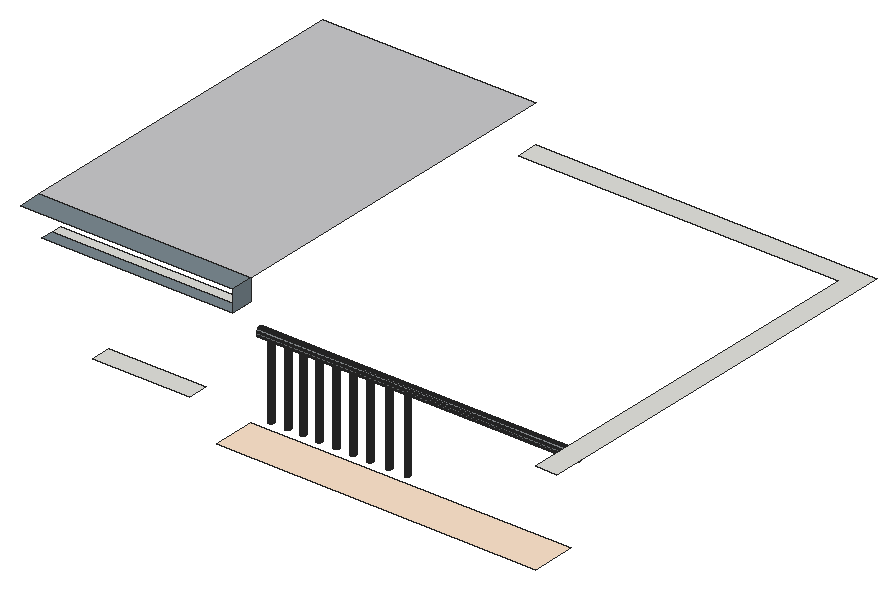
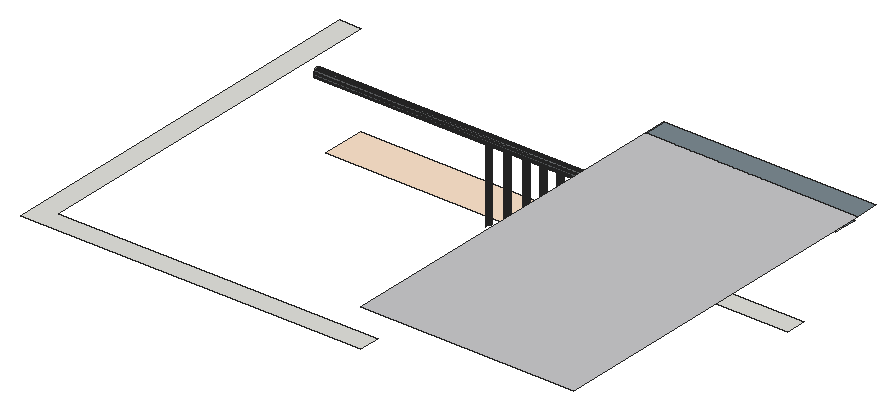
# SketchUp Ruby script. Lengths in inches.
U = 1.inch
M = Sketchup.active_model
def pt(a) = Geom::Point3d.new(a.map { |v| v * U })
def face(e, loops, mat)
  f = e.add_face(loops[0].map { |a| pt(a) })
  loops[1..].each { |l| e.add_face(l.map { |a| pt(a) }).erase! }
  f.material = f.back_material = mat if mat
  f
end
# faces: each face lists its corners as indices into pts; further lists are holes
def faces(e, pts, list, mat = nil) = list.each { |f| face(e, (f[0].is_a?(Array) ? f : [f]).map { |l| l.map { |i| pts[i] } }, mat) }
# xy, xz, yz: faces in a plane at the given z, y or x. An outline is a flat list of corners, or four numbers for a rectangle; further outlines are holes
def ring(l) = l.size == 4 ? [[l[0], l[1]], [l[2], l[1]], [l[2], l[3]], [l[0], l[3]]] : l.each_slice(2).to_a
def flat(e, list, mat, &to3) = list.each { |f| face(e, (f[0].is_a?(Array) ? f : [f]).map { |l| ring(l).map { |u, v| to3.(u, v) } }, mat) }
def xy(e, z, list, mat = nil) = flat(e, list, mat) { |x, y| [x, y, z] }
def xz(e, y, list, mat = nil) = flat(e, list, mat) { |x, z| [x, y, z] }
def yz(e, x, list, mat = nil) = flat(e, list, mat) { |y, z| [x, y, z] }
def lines(e, pts, list) = list.each { |a, b| e.add_line(pt(pts[a]), pt(pts[b])) }
# prism: a flat outline (further loops are holes) pulled along v
def prism(e, loops, v, mat = nil)
  f = face(e, loops, mat); d = Geom::Vector3d.new(v.map { |x| x * U })
  f.pushpull(f.normal.samedirection?(d) ? d.length : -d.length)
end
def box(e, o, s, mat = nil) = prism(e, [[o, [o[0] + s[0], o[1], o[2]], [o[0] + s[0], o[1] + s[1], o[2]], [o[0], o[1] + s[1], o[2]]]], [0, 0, s[2]], mat)
def at(x, y, z, deg = 0) = Geom::Transformation.translation(pt([x, y, z])) * Geom::Transformation.rotation(ORIGIN, Z_AXIS, deg.degrees)
def axes(o, x, y, z) = Geom::Transformation.new([*x, 0, *y, 0, *z, 0, *pt(o).to_a, 1])
def part(name) = M.definitions.add(name)
# library, detail: a bought-in or finely detailed component or shape, given as its bounding box
def library(name, o, s) = part(name).tap { |d| box(d.entities, o, s) }
def detail(e, o, s) = box(e.add_group.entities, o, s)
def put(e, d, t, mat = nil) = e.add_instance(d, t).tap { |i| i.material = mat if mat }
def group(e, t, mat = nil) = e.add_group.tap { |g| g.transformation = t; g.material = mat if mat }.entities
root = M.entities
M.materials.add("[Blacktop Old 01]").color = [132, 136, 139]
M.materials.add("[Color C01]").color = [255, 229, 204]
M.materials.add("[Formica Speckled Grey]").color = [123, 137, 145]
M.materials.add("[Polished Concrete New]").color = [200, 200, 203]
M.materials.add("[Terrazzo Light Blue]").color = [196, 214, 227]
xy(root,2196.1875,[[746.18,617.28,1870.17,769.97]],"[Color C01]")
xy(root,2229.35,[[218.87,733.78,559.3,805.03]])
xy(root,2459.4375,[[1199.35,798.92,1201.92,799.26,1204.32,800.25,1206.375,801.83,1207.95,803.89,1208.95,806.29,1209.29,808.86,1208.95,811.43,1207.95,813.83,1206.375,815.89,1204.32,817.46,1201.92,818.46,1199.35,818.8,1196.78,818.46,1194.38,817.46,1192.32,815.89,1190.74,813.83,1189.75,811.43,1189.41,808.86,1189.75,806.29,1190.74,803.89,1192.32,801.83,1194.38,800.25,1196.78,799.26]])
xy(root,2460.4375,[[1524.85,798.92,1527.42,799.26,1529.82,800.25,1531.875,801.83,1533.45,803.89,1534.45,806.29,1534.79,808.86,1534.45,811.43,1533.45,813.83,1531.875,815.89,1529.82,817.46,1527.42,818.46,1524.85,818.8,1522.28,818.46,1519.88,817.46,1517.82,815.89,1516.24,813.83,1515.25,811.43,1514.91,808.86,1515.25,806.29,1516.24,803.89,1517.82,801.83,1519.88,800.25,1522.28,799.26]])
xy(root,2461.125,[[1396.47,798.92,1399.05,799.26,1401.44,800.25,1403.5,801.83,1405.08,803.89,1406.07,806.29,1406.41,808.86,1406.07,811.43,1405.08,813.83,1403.5,815.89,1401.44,817.46,1399.05,818.46,1396.47,818.8,1393.9,818.46,1391.5,817.46,1389.45,815.89,1387.87,813.83,1386.875,811.43,1386.54,808.86,1386.875,806.29,1387.87,803.89,1389.45,801.83,1391.5,800.25,1393.9,799.26]])
xy(root,2462.0625,[[954.66,798.92,957.23,799.26,959.63,800.25,961.6875,801.83,963.27,803.89,964.26,806.29,964.6,808.86,964.26,811.43,963.27,813.83,961.6875,815.89,959.63,817.46,957.23,818.46,954.66,818.8,952.09,818.46,949.69,817.46,947.63,815.89,946.06,813.83,945.0625,811.43,944.72,808.86,945.0625,806.29,946.06,803.89,947.63,801.83,949.69,800.25,952.09,799.26]])
xy(root,2462.1875,[[1135.1,798.92,1137.67,799.26,1140.07,800.25,1142.125,801.83,1143.7,803.89,1144.7,806.29,1145.04,808.86,1144.7,811.43,1143.7,813.83,1142.125,815.89,1140.07,817.46,1137.67,818.46,1135.1,818.8,1132.53,818.46,1130.13,817.46,1128.07,815.89,1126.49,813.83,1125.5,811.43,1125.16,808.86,1125.5,806.29,1126.49,803.89,1128.07,801.83,1130.13,800.25,1132.53,799.26]])
xy(root,2464.4375,[[1644.29,798.92,1646.86,799.26,1649.25,800.25,1651.3125,801.83,1652.89,803.89,1653.89,806.29,1654.22,808.86,1653.89,811.43,1652.89,813.83,1651.3125,815.89,1649.25,817.46,1646.86,818.46,1644.29,818.8,1641.71,818.46,1639.32,817.46,1637.26,815.89,1635.68,813.83,1634.6875,811.43,1634.35,808.86,1634.6875,806.29,1635.68,803.89,1637.26,801.83,1639.32,800.25,1641.71,799.26]])
xy(root,2464.74,[[1015.1,798.92,1017.67,799.26,1020.07,800.25,1022.125,801.83,1023.7,803.89,1024.7,806.29,1025.04,808.86,1024.7,811.43,1023.7,813.83,1022.125,815.89,1020.07,817.46,1017.67,818.46,1015.1,818.8,1012.53,818.46,1010.13,817.46,1008.07,815.89,1006.49,813.83,1005.5,811.43,1005.16,808.86,1005.5,806.29,1006.49,803.89,1008.07,801.83,1010.13,800.25,1012.53,799.26],[1760.72,798.92,1763.3,799.26,1765.69,800.25,1767.75,801.83,1769.33,803.89,1770.32,806.29,1770.66,808.86,1770.32,811.43,1769.33,813.83,1767.75,815.89,1765.69,817.46,1763.3,818.46,1760.72,818.8,1758.15,818.46,1755.75,817.46,1753.7,815.89,1752.12,813.83,1751.125,811.43,1750.79,808.86,1751.125,806.29,1752.12,803.89,1753.7,801.83,1755.75,800.25,1758.15,799.26]])
xy(root,2466.1875,[[1705.97,798.92,1708.55,799.26,1710.94,800.25,1713,801.83,1714.58,803.89,1715.57,806.29,1715.91,808.86,1715.57,811.43,1714.58,813.83,1713,815.89,1710.94,817.46,1708.55,818.46,1705.97,818.8,1703.4,818.46,1701,817.46,1698.95,815.89,1697.37,813.83,1696.375,811.43,1696.04,808.86,1696.375,806.29,1697.37,803.89,1698.95,801.83,1701,800.25,1703.4,799.26]])
xy(root,2467.625,[[845.1,798.92,847.67,799.26,850.07,800.25,852.125,801.83,853.7,803.89,854.7,806.29,855.04,808.86,854.7,811.43,853.7,813.83,852.125,815.89,850.07,817.46,847.67,818.46,845.1,818.8,842.53,818.46,840.13,817.46,838.07,815.89,836.49,813.83,835.5,811.43,835.16,808.86,835.5,806.29,836.49,803.89,838.07,801.83,840.13,800.25,842.53,799.26]])
xy(root,2468.78,[[785.04,798.92,787.61,799.26,790,800.25,792.0625,801.83,793.64,803.89,794.64,806.29,794.97,808.86,794.64,811.43,793.64,813.83,792.0625,815.89,790,817.46,787.61,818.46,785.04,818.8,782.46,818.46,780.07,817.46,778.01,815.89,776.43,813.83,775.4375,811.43,775.1,808.86,775.4375,806.29,776.43,803.89,778.01,801.83,780.07,800.25,782.46,799.26],[1263.54,798.92,1266.11,799.26,1268.5,800.25,1270.5625,801.83,1272.14,803.89,1273.14,806.29,1273.47,808.86,1273.14,811.43,1272.14,813.83,1270.5625,815.89,1268.5,817.46,1266.11,818.46,1263.54,818.8,1260.96,818.46,1258.57,817.46,1256.51,815.89,1254.93,813.83,1253.9375,811.43,1253.6,808.86,1253.9375,806.29,1254.93,803.89,1256.51,801.83,1258.57,800.25,1260.96,799.26],[1461.66,798.92,1464.23,799.26,1466.63,800.25,1468.6875,801.83,1470.27,803.89,1471.26,806.29,1471.6,808.86,1471.26,811.43,1470.27,813.83,1468.6875,815.89,1466.63,817.46,1464.23,818.46,1461.66,818.8,1459.09,818.46,1456.69,817.46,1454.63,815.89,1453.06,813.83,1452.0625,811.43,1451.72,808.86,1452.0625,806.29,1453.06,803.89,1454.63,801.83,1456.69,800.25,1459.09,799.26]])
xy(root,2472.82,[[898.66,798.92,901.23,799.26,903.63,800.25,905.6875,801.83,907.27,803.89,908.26,806.29,908.6,808.86,908.26,811.43,907.27,813.83,905.6875,815.89,903.63,817.46,901.23,818.46,898.66,818.8,896.09,818.46,893.69,817.46,891.63,815.89,890.06,813.83,889.0625,811.43,888.72,808.86,889.0625,806.29,890.06,803.89,891.63,801.83,893.69,800.25,896.09,799.26],[1332.66,798.92,1335.23,799.26,1337.63,800.25,1339.6875,801.83,1341.27,803.89,1342.26,806.29,1342.6,808.86,1342.26,811.43,1341.27,813.83,1339.6875,815.89,1337.63,817.46,1335.23,818.46,1332.66,818.8,1330.09,818.46,1327.69,817.46,1325.63,815.89,1324.06,813.83,1323.0625,811.43,1322.72,808.86,1323.0625,806.29,1324.06,803.89,1325.63,801.83,1327.69,800.25,1330.09,799.26],[1581.79,798.92,1584.36,799.26,1586.75,800.25,1588.8125,801.83,1590.39,803.89,1591.39,806.29,1591.72,808.86,1591.39,811.43,1590.39,813.83,1588.8125,815.89,1586.75,817.46,1584.36,818.46,1581.79,818.8,1579.21,818.46,1576.82,817.46,1574.76,815.89,1573.18,813.83,1572.1875,811.43,1571.85,808.86,1572.1875,806.29,1573.18,803.89,1574.76,801.83,1576.82,800.25,1579.21,799.26]])
xy(root,2472.9375,[[1818.72,798.92,1821.3,799.26,1823.69,800.25,1825.75,801.83,1827.33,803.89,1828.32,806.29,1828.66,808.86,1828.32,811.43,1827.33,813.83,1825.75,815.89,1823.69,817.46,1821.3,818.46,1818.72,818.8,1816.15,818.46,1813.75,817.46,1811.7,815.89,1810.12,813.83,1809.125,811.43,1808.79,808.86,1809.125,806.29,1810.12,803.89,1811.7,801.83,1813.75,800.25,1816.15,799.26]])
xy(root,2473.4375,[[1074.1,798.92,1076.67,799.26,1079.07,800.25,1081.125,801.83,1082.7,803.89,1083.7,806.29,1084.04,808.86,1083.7,811.43,1082.7,813.83,1081.125,815.89,1079.07,817.46,1076.67,818.46,1074.1,818.8,1071.53,818.46,1069.13,817.46,1067.07,815.89,1065.49,813.83,1064.5,811.43,1064.16,808.86,1064.5,806.29,1065.49,803.89,1067.07,801.83,1069.13,800.25,1071.53,799.26]])
xy(root,2522.1875,[[1870.17,617.28,1944.31,617.28,1944.31,2018.8,746.18,2018.8,746.18,1944.66,1870.17,1944.66]])
xy(root,2578.28,[[77.12,733.78,746.18,769.97]])
xy(root,2578.28,[[77.12,688.65,746.18,733.78]],"[Formica Speckled Grey]")
xy(root,2654.3125,[[0,688.65,746.18,769.97]],"[Formica Speckled Grey]")
xy(root,2654.3125,[[0,769.97,746.18,2018.8]],"[Polished Concrete New]")
yz(root,746.18,[[688.65,2578.28,769.97,2654.3125]],"[Formica Speckled Grey]")
yz(root,1870.17,[[808.34,2453.16,812.38,2453.6875,816.15,2455.25,819.39,2457.73,821.87,2460.97,823.43,2464.74,823.96,2468.78,823.43,2472.82,821.87,2476.59,819.39,2479.83,816.15,2482.3125,812.38,2483.875,808.34,2484.41,804.29,2483.875,800.53,2482.3125,797.29,2479.83,794.81,2476.59,793.25,2472.82,792.71,2468.78,793.25,2464.74,794.81,2460.97,797.29,2457.73,800.53,2455.25,804.29,2453.6875]])
p = [[782.46,799.26,2196.1875],[785.04,798.92,2196.1875],[785.04,798.92,2468.78],[782.46,799.26,2468.78],[787.61,799.26,2196.1875],[787.61,799.26,2468.78],
  [842.53,799.26,2196.1875],[845.1,798.92,2196.1875],[845.1,798.92,2467.625],[842.53,799.26,2467.625],[847.67,799.26,2196.1875],[847.67,799.26,2467.625],
  [896.09,799.26,2196.1875],[898.66,798.92,2196.1875],[898.66,798.92,2472.82],[896.09,799.26,2472.82],[901.23,799.26,2196.1875],[901.23,799.26,2472.82],
  [952.09,799.26,2196.1875],[954.66,798.92,2196.1875],[954.66,798.92,2462.0625],[952.09,799.26,2462.0625],[957.23,799.26,2196.1875],[957.23,799.26,2462.0625],
  [1012.53,799.26,2196.1875],[1015.1,798.92,2196.1875],[1015.1,798.92,2464.74],[1012.53,799.26,2464.74],[1017.67,799.26,2196.1875],[1017.67,799.26,2464.74],
  [1071.53,799.26,2196.1875],[1074.1,798.92,2196.1875],[1074.1,798.92,2473.4375],[1071.53,799.26,2473.4375],[1076.67,799.26,2196.1875],[1076.67,799.26,2473.4375],
  [1132.53,799.26,2196.1875],[1135.1,798.92,2196.1875],[1135.1,798.92,2462.1875],[1132.53,799.26,2462.1875],[1137.67,799.26,2196.1875],[1137.67,799.26,2462.1875],
  [1196.78,799.26,2196.1875],[1199.35,798.92,2196.1875],[1199.35,798.92,2459.4375],[1196.78,799.26,2459.4375],[1201.92,799.26,2196.1875],[1201.92,799.26,2459.4375],
  [1263.54,798.92,2196.1875],[1266.11,799.26,2196.1875],[1266.11,799.26,2468.78],[1263.54,798.92,2468.78],[780.07,800.25,2196.1875],[780.07,800.25,2468.78],
  [790,800.25,2196.1875],[790,800.25,2468.78],[840.13,800.25,2196.1875],[840.13,800.25,2467.625],[850.07,800.25,2196.1875],[850.07,800.25,2467.625],
  [893.69,800.25,2196.1875],[893.69,800.25,2472.82],[903.63,800.25,2196.1875],[903.63,800.25,2472.82],[949.69,800.25,2196.1875],[949.69,800.25,2462.0625],
  [959.63,800.25,2196.1875],[959.63,800.25,2462.0625],[1010.13,800.25,2196.1875],[1010.13,800.25,2464.74],[1020.07,800.25,2196.1875],[1020.07,800.25,2464.74],
  [1069.13,800.25,2196.1875],[1069.13,800.25,2473.4375],[1079.07,800.25,2196.1875],[1079.07,800.25,2473.4375],[1130.13,800.25,2196.1875],[1130.13,800.25,2462.1875],
  [1140.07,800.25,2196.1875],[1140.07,800.25,2462.1875],[1194.38,800.25,2196.1875],[1194.38,800.25,2459.4375],[1204.32,800.25,2196.1875],[1204.32,800.25,2459.4375],
  [1268.5,800.25,2196.1875],[1268.5,800.25,2468.78],[778.01,801.83,2196.1875],[778.01,801.83,2468.78],[792.0625,801.83,2196.1875],[792.0625,801.83,2468.78],
  [838.07,801.83,2196.1875],[838.07,801.83,2467.625],[852.125,801.83,2196.1875],[852.125,801.83,2467.625],[891.63,801.83,2196.1875],[891.63,801.83,2472.82],
  [905.6875,801.83,2196.1875],[905.6875,801.83,2472.82],[947.63,801.83,2196.1875],[947.63,801.83,2462.0625],[961.6875,801.83,2196.1875],[961.6875,801.83,2462.0625],
  [1008.07,801.83,2196.1875],[1008.07,801.83,2464.74],[1022.125,801.83,2196.1875],[1022.125,801.83,2464.74],[1067.07,801.83,2196.1875],[1067.07,801.83,2473.4375],
  [1081.125,801.83,2196.1875],[1081.125,801.83,2473.4375],[1128.07,801.83,2196.1875],[1128.07,801.83,2462.1875],[1142.125,801.83,2196.1875],[1142.125,801.83,2462.1875],
  [1192.32,801.83,2196.1875],[1192.32,801.83,2459.4375],[1206.375,801.83,2196.1875],[1206.375,801.83,2459.4375],[1270.5625,801.83,2196.1875],[1270.5625,801.83,2468.78],
  [776.43,803.89,2196.1875],[776.43,803.89,2468.78],[793.64,803.89,2196.1875],[793.64,803.89,2468.78],[836.49,803.89,2196.1875],[836.49,803.89,2467.625],
  [853.7,803.89,2196.1875],[853.7,803.89,2467.625],[890.06,803.89,2196.1875],[890.06,803.89,2472.82],[907.27,803.89,2196.1875],[907.27,803.89,2472.82],
  [946.06,803.89,2196.1875],[946.06,803.89,2462.0625],[963.27,803.89,2196.1875],[963.27,803.89,2462.0625],[1006.49,803.89,2196.1875],[1006.49,803.89,2464.74],
  [1023.7,803.89,2196.1875],[1023.7,803.89,2464.74],[1065.49,803.89,2196.1875],[1065.49,803.89,2473.4375],[1082.7,803.89,2196.1875],[1082.7,803.89,2473.4375],
  [1126.49,803.89,2196.1875],[1126.49,803.89,2462.1875],[1143.7,803.89,2196.1875],[1143.7,803.89,2462.1875],[1190.74,803.89,2196.1875],[1190.74,803.89,2459.4375],
  [1207.95,803.89,2196.1875],[1207.95,803.89,2459.4375],[1272.14,803.89,2196.1875],[1272.14,803.89,2468.78],[775.4375,806.29,2196.1875],[775.4375,806.29,2468.78],
  [794.64,806.29,2196.1875],[794.64,806.29,2468.78],[835.5,806.29,2196.1875],[835.5,806.29,2467.625],[854.7,806.29,2196.1875],[854.7,806.29,2467.625],
  [889.0625,806.29,2196.1875],[889.0625,806.29,2472.82],[908.26,806.29,2196.1875],[908.26,806.29,2472.82],[945.0625,806.29,2196.1875],[945.0625,806.29,2462.0625],
  [964.26,806.29,2196.1875],[964.26,806.29,2462.0625],[1005.5,806.29,2196.1875],[1005.5,806.29,2464.74],[1024.7,806.29,2196.1875],[1024.7,806.29,2464.74],
  [1064.5,806.29,2196.1875],[1064.5,806.29,2473.4375],[1083.7,806.29,2196.1875],[1083.7,806.29,2473.4375],[1125.5,806.29,2196.1875],[1125.5,806.29,2462.1875],
  [1144.7,806.29,2196.1875],[1144.7,806.29,2462.1875],[1189.75,806.29,2196.1875],[1189.75,806.29,2459.4375],[1208.95,806.29,2196.1875],[1208.95,806.29,2459.4375],
  [1273.14,806.29,2196.1875],[1273.14,806.29,2468.78],[775.1,808.86,2196.1875],[775.1,808.86,2468.78],[794.97,808.86,2196.1875],[794.97,808.86,2468.78],
  [835.16,808.86,2196.1875],[835.16,808.86,2467.625],[855.04,808.86,2196.1875],[855.04,808.86,2467.625],[888.72,808.86,2196.1875],[888.72,808.86,2472.82],
  [908.6,808.86,2196.1875],[908.6,808.86,2472.82],[944.72,808.86,2196.1875],[944.72,808.86,2462.0625],[964.6,808.86,2196.1875],[964.6,808.86,2462.0625],
  [1005.16,808.86,2196.1875],[1005.16,808.86,2464.74],[1025.04,808.86,2196.1875],[1025.04,808.86,2464.74],[1064.16,808.86,2196.1875],[1064.16,808.86,2473.4375],
  [1084.04,808.86,2196.1875],[1084.04,808.86,2473.4375],[1125.16,808.86,2196.1875],[1125.16,808.86,2462.1875],[1145.04,808.86,2196.1875],[1145.04,808.86,2462.1875],
  [1189.41,808.86,2196.1875],[1189.41,808.86,2459.4375],[1209.29,808.86,2196.1875],[1209.29,808.86,2459.4375],[1273.47,808.86,2196.1875],[1273.47,808.86,2468.78],
  [775.4375,811.43,2196.1875],[775.4375,811.43,2468.78],[794.64,811.43,2196.1875],[794.64,811.43,2468.78],[835.5,811.43,2196.1875],[835.5,811.43,2467.625],
  [854.7,811.43,2196.1875],[854.7,811.43,2467.625],[889.0625,811.43,2196.1875],[889.0625,811.43,2472.82],[908.26,811.43,2196.1875],[908.26,811.43,2472.82],
  [945.0625,811.43,2196.1875],[945.0625,811.43,2462.0625],[964.26,811.43,2196.1875],[964.26,811.43,2462.0625],[1005.5,811.43,2196.1875],[1005.5,811.43,2464.74],
  [1024.7,811.43,2196.1875],[1024.7,811.43,2464.74],[1064.5,811.43,2196.1875],[1064.5,811.43,2473.4375],[1083.7,811.43,2196.1875],[1083.7,811.43,2473.4375],
  [1125.5,811.43,2196.1875],[1125.5,811.43,2462.1875],[1144.7,811.43,2196.1875],[1144.7,811.43,2462.1875],[1189.75,811.43,2196.1875],[1189.75,811.43,2459.4375],
  [1208.95,811.43,2196.1875],[1208.95,811.43,2459.4375],[1273.14,811.43,2196.1875],[1273.14,811.43,2468.78],[776.43,813.83,2196.1875],[776.43,813.83,2468.78],
  [793.64,813.83,2196.1875],[793.64,813.83,2468.78],[836.49,813.83,2196.1875],[836.49,813.83,2467.625],[853.7,813.83,2196.1875],[853.7,813.83,2467.625],
  [890.06,813.83,2196.1875],[890.06,813.83,2472.82],[907.27,813.83,2196.1875],[907.27,813.83,2472.82],[946.06,813.83,2196.1875],[946.06,813.83,2462.0625],
  [963.27,813.83,2196.1875],[963.27,813.83,2462.0625],[1006.49,813.83,2196.1875],[1006.49,813.83,2464.74],[1023.7,813.83,2196.1875],[1023.7,813.83,2464.74],
  [1065.49,813.83,2196.1875],[1065.49,813.83,2473.4375],[1082.7,813.83,2196.1875],[1082.7,813.83,2473.4375],[1126.49,813.83,2196.1875],[1126.49,813.83,2462.1875],
  [1143.7,813.83,2196.1875],[1143.7,813.83,2462.1875],[1190.74,813.83,2196.1875],[1190.74,813.83,2459.4375],[1207.95,813.83,2196.1875],[1207.95,813.83,2459.4375],
  [1272.14,813.83,2196.1875],[1272.14,813.83,2468.78],[778.01,815.89,2196.1875],[778.01,815.89,2468.78],[792.0625,815.89,2196.1875],[792.0625,815.89,2468.78],
  [838.07,815.89,2196.1875],[838.07,815.89,2467.625],[852.125,815.89,2196.1875],[852.125,815.89,2467.625],[891.63,815.89,2196.1875],[891.63,815.89,2472.82],
  [905.6875,815.89,2196.1875],[905.6875,815.89,2472.82],[947.63,815.89,2196.1875],[947.63,815.89,2462.0625],[961.6875,815.89,2196.1875],[961.6875,815.89,2462.0625],
  [1008.07,815.89,2196.1875],[1008.07,815.89,2464.74],[1022.125,815.89,2196.1875],[1022.125,815.89,2464.74],[1067.07,815.89,2196.1875],[1067.07,815.89,2473.4375],
  [1081.125,815.89,2196.1875],[1081.125,815.89,2473.4375],[1128.07,815.89,2196.1875],[1128.07,815.89,2462.1875],[1142.125,815.89,2196.1875],[1142.125,815.89,2462.1875],
  [1192.32,815.89,2196.1875],[1192.32,815.89,2459.4375],[1206.375,815.89,2196.1875],[1206.375,815.89,2459.4375],[1270.5625,815.89,2196.1875],[1270.5625,815.89,2468.78],
  [780.07,817.46,2196.1875],[780.07,817.46,2468.78],[790,817.46,2196.1875],[790,817.46,2468.78],[840.13,817.46,2196.1875],[840.13,817.46,2467.625],
  [850.07,817.46,2196.1875],[850.07,817.46,2467.625],[893.69,817.46,2196.1875],[893.69,817.46,2472.82],[903.63,817.46,2196.1875],[903.63,817.46,2472.82],
  [949.69,817.46,2196.1875],[949.69,817.46,2462.0625],[959.63,817.46,2196.1875],[959.63,817.46,2462.0625],[1010.13,817.46,2196.1875],[1010.13,817.46,2464.74],
  [1020.07,817.46,2196.1875],[1020.07,817.46,2464.74],[1069.13,817.46,2196.1875],[1069.13,817.46,2473.4375],[1079.07,817.46,2196.1875],[1079.07,817.46,2473.4375],
  [1130.13,817.46,2196.1875],[1130.13,817.46,2462.1875],[1140.07,817.46,2196.1875],[1140.07,817.46,2462.1875],[1194.38,817.46,2196.1875],[1194.38,817.46,2459.4375],
  [1204.32,817.46,2196.1875],[1204.32,817.46,2459.4375],[782.46,818.46,2196.1875],[782.46,818.46,2468.78],[787.61,818.46,2196.1875],[787.61,818.46,2468.78],
  [842.53,818.46,2196.1875],[842.53,818.46,2467.625],[847.67,818.46,2196.1875],[847.67,818.46,2467.625],[896.09,818.46,2196.1875],[896.09,818.46,2472.82],
  [901.23,818.46,2196.1875],[901.23,818.46,2472.82],[952.09,818.46,2196.1875],[952.09,818.46,2462.0625],[957.23,818.46,2196.1875],[957.23,818.46,2462.0625],
  [1012.53,818.46,2196.1875],[1012.53,818.46,2464.74],[1017.67,818.46,2196.1875],[1017.67,818.46,2464.74],[1071.53,818.46,2196.1875],[1071.53,818.46,2473.4375],
  [1076.67,818.46,2196.1875],[1076.67,818.46,2473.4375],[1132.53,818.46,2196.1875],[1132.53,818.46,2462.1875],[1137.67,818.46,2196.1875],[1137.67,818.46,2462.1875],
  [1196.78,818.46,2196.1875],[1196.78,818.46,2459.4375],[1201.92,818.46,2196.1875],[1201.92,818.46,2459.4375],[785.04,818.8,2196.1875],[785.04,818.8,2468.78],
  [845.1,818.8,2196.1875],[845.1,818.8,2467.625],[898.66,818.8,2196.1875],[898.66,818.8,2472.82],[954.66,818.8,2196.1875],[954.66,818.8,2462.0625],
  [1015.1,818.8,2196.1875],[1015.1,818.8,2464.74],[1074.1,818.8,2196.1875],[1074.1,818.8,2473.4375],[1135.1,818.8,2196.1875],[1135.1,818.8,2462.1875],
  [1199.35,818.8,2196.1875],[1199.35,818.8,2459.4375],[1870.17,808.34,2453.16],[1870.17,804.29,2453.6875],[746.18,804.29,2453.6875],[746.18,808.34,2453.16],
  [1870.17,812.38,2453.6875],[746.18,812.38,2453.6875],[1870.17,800.53,2455.25],[746.18,800.53,2455.25],[1870.17,816.15,2455.25],[746.18,816.15,2455.25],
  [1870.17,797.29,2457.73],[746.18,797.29,2457.73],[1870.17,819.39,2457.73],[746.18,819.39,2457.73],[1870.17,794.81,2460.97],[746.18,794.81,2460.97],
  [1870.17,821.87,2460.97],[746.18,821.87,2460.97],[1870.17,793.25,2464.74],[746.18,793.25,2464.74],[1870.17,823.43,2464.74],[746.18,823.43,2464.74],
  [1870.17,792.71,2468.78],[746.18,792.71,2468.78],[1870.17,823.96,2468.78],[746.18,823.96,2468.78],[1870.17,793.25,2472.82],[746.18,793.25,2472.82],
  [1870.17,823.43,2472.82],[746.18,823.43,2472.82],[1870.17,794.81,2476.59],[746.18,794.81,2476.59],[1870.17,821.87,2476.59],[746.18,821.87,2476.59],
  [1870.17,797.29,2479.83],[746.18,797.29,2479.83],[1870.17,819.39,2479.83],[746.18,819.39,2479.83],[1870.17,800.53,2482.3125],[746.18,800.53,2482.3125],
  [1870.17,816.15,2482.3125],[746.18,816.15,2482.3125],[1870.17,804.29,2483.875],[746.18,804.29,2483.875],[1870.17,812.38,2483.875],[746.18,812.38,2483.875],
  [1870.17,808.34,2484.41],[746.18,808.34,2484.41]]
faces(root,p,[[0,1,2,3],[1,4,5,2],[6,7,8,9],[7,10,11,8],[12,13,14,15],[13,16,17,14],[18,19,20,21],[19,22,23,20],
  [24,25,26,27],[25,28,29,26],[30,31,32,33],[31,34,35,32],[36,37,38,39],[37,40,41,38],[42,43,44,45],[43,46,47,44],
  [48,49,50,51],[52,0,3,53],[4,54,55,5],[56,6,9,57],[10,58,59,11],[60,12,15,61],[16,62,63,17],[64,18,21,65],
  [22,66,67,23],[68,24,27,69],[28,70,71,29],[72,30,33,73],[34,74,75,35],[76,36,39,77],[40,78,79,41],[80,42,45,81],
  [46,82,83,47],[49,84,85,50],[86,52,53,87],[54,88,89,55],[90,56,57,91],[58,92,93,59],[94,60,61,95],[62,96,97,63],
  [98,64,65,99],[66,100,101,67],[102,68,69,103],[70,104,105,71],[106,72,73,107],[74,108,109,75],[110,76,77,111],[78,112,113,79],
  [114,80,81,115],[82,116,117,83],[84,118,119,85],[120,86,87,121],[88,122,123,89],[124,90,91,125],[92,126,127,93],[128,94,95,129],
  [96,130,131,97],[132,98,99,133],[100,134,135,101],[136,102,103,137],[104,138,139,105],[140,106,107,141],[108,142,143,109],[144,110,111,145],
  [112,146,147,113],[148,114,115,149],[116,150,151,117],[118,152,153,119],[154,120,121,155],[122,156,157,123],[158,124,125,159],[126,160,161,127],
  [162,128,129,163],[130,164,165,131],[166,132,133,167],[134,168,169,135],[170,136,137,171],[138,172,173,139],[174,140,141,175],[142,176,177,143],
  [178,144,145,179],[146,180,181,147],[182,148,149,183],[150,184,185,151],[152,186,187,153],[188,154,155,189],[156,190,191,157],[192,158,159,193],
  [160,194,195,161],[196,162,163,197],[164,198,199,165],[200,166,167,201],[168,202,203,169],[204,170,171,205],[172,206,207,173],[208,174,175,209],
  [176,210,211,177],[212,178,179,213],[180,214,215,181],[216,182,183,217],[184,218,219,185],[186,220,221,187],[222,188,189,223],[190,224,225,191],
  [226,192,193,227],[194,228,229,195],[230,196,197,231],[198,232,233,199],[234,200,201,235],[202,236,237,203],[238,204,205,239],[206,240,241,207],
  [242,208,209,243],[210,244,245,211],[246,212,213,247],[214,248,249,215],[250,216,217,251],[218,252,253,219],[220,254,255,221],[256,222,223,257],
  [224,258,259,225],[260,226,227,261],[228,262,263,229],[264,230,231,265],[232,266,267,233],[268,234,235,269],[236,270,271,237],[272,238,239,273],
  [240,274,275,241],[276,242,243,277],[244,278,279,245],[280,246,247,281],[248,282,283,249],[284,250,251,285],[252,286,287,253],[254,288,289,255],
  [290,256,257,291],[258,292,293,259],[294,260,261,295],[262,296,297,263],[298,264,265,299],[266,300,301,267],[302,268,269,303],[270,304,305,271],
  [306,272,273,307],[274,308,309,275],[310,276,277,311],[278,312,313,279],[314,280,281,315],[282,316,317,283],[318,284,285,319],[286,320,321,287],
  [288,322,323,289],[324,290,291,325],[292,326,327,293],[328,294,295,329],[296,330,331,297],[332,298,299,333],[300,334,335,301],[336,302,303,337],
  [304,338,339,305],[340,306,307,341],[308,342,343,309],[344,310,311,345],[312,346,347,313],[348,314,315,349],[316,350,351,317],[352,318,319,353],
  [320,354,355,321],[356,324,325,357],[326,358,359,327],[360,328,329,361],[330,362,363,331],[364,332,333,365],[334,366,367,335],[368,336,337,369],
  [338,370,371,339],[372,340,341,373],[342,374,375,343],[376,344,345,377],[346,378,379,347],[380,348,349,381],[350,382,383,351],[384,352,353,385],
  [354,386,387,355],[388,356,357,389],[358,388,389,359],[390,360,361,391],[362,390,391,363],[392,364,365,393],[366,392,393,367],[394,368,369,395],
  [370,394,395,371],[396,372,373,397],[374,396,397,375],[398,376,377,399],[378,398,399,379],[400,380,381,401],[382,400,401,383],[402,384,385,403],
  [386,402,403,387]],"[Terrazzo Light Blue]")
faces(root,p,[[404,405,406,407],[408,404,407,409],[405,410,411,406],[412,408,409,413],[410,414,415,411],[416,412,413,417],[414,418,419,415],[420,416,417,421],
  [418,422,423,419],[424,420,421,425],[422,426,427,423],[428,424,425,429],[426,430,431,427],[432,428,429,433],[430,434,435,431],[436,432,433,437],
  [434,438,439,435],[440,436,437,441],[438,442,443,439],[444,440,441,445],[442,446,447,443],[448,444,445,449],[446,450,451,447],[450,448,449,451]],"[Blacktop Old 01]")
